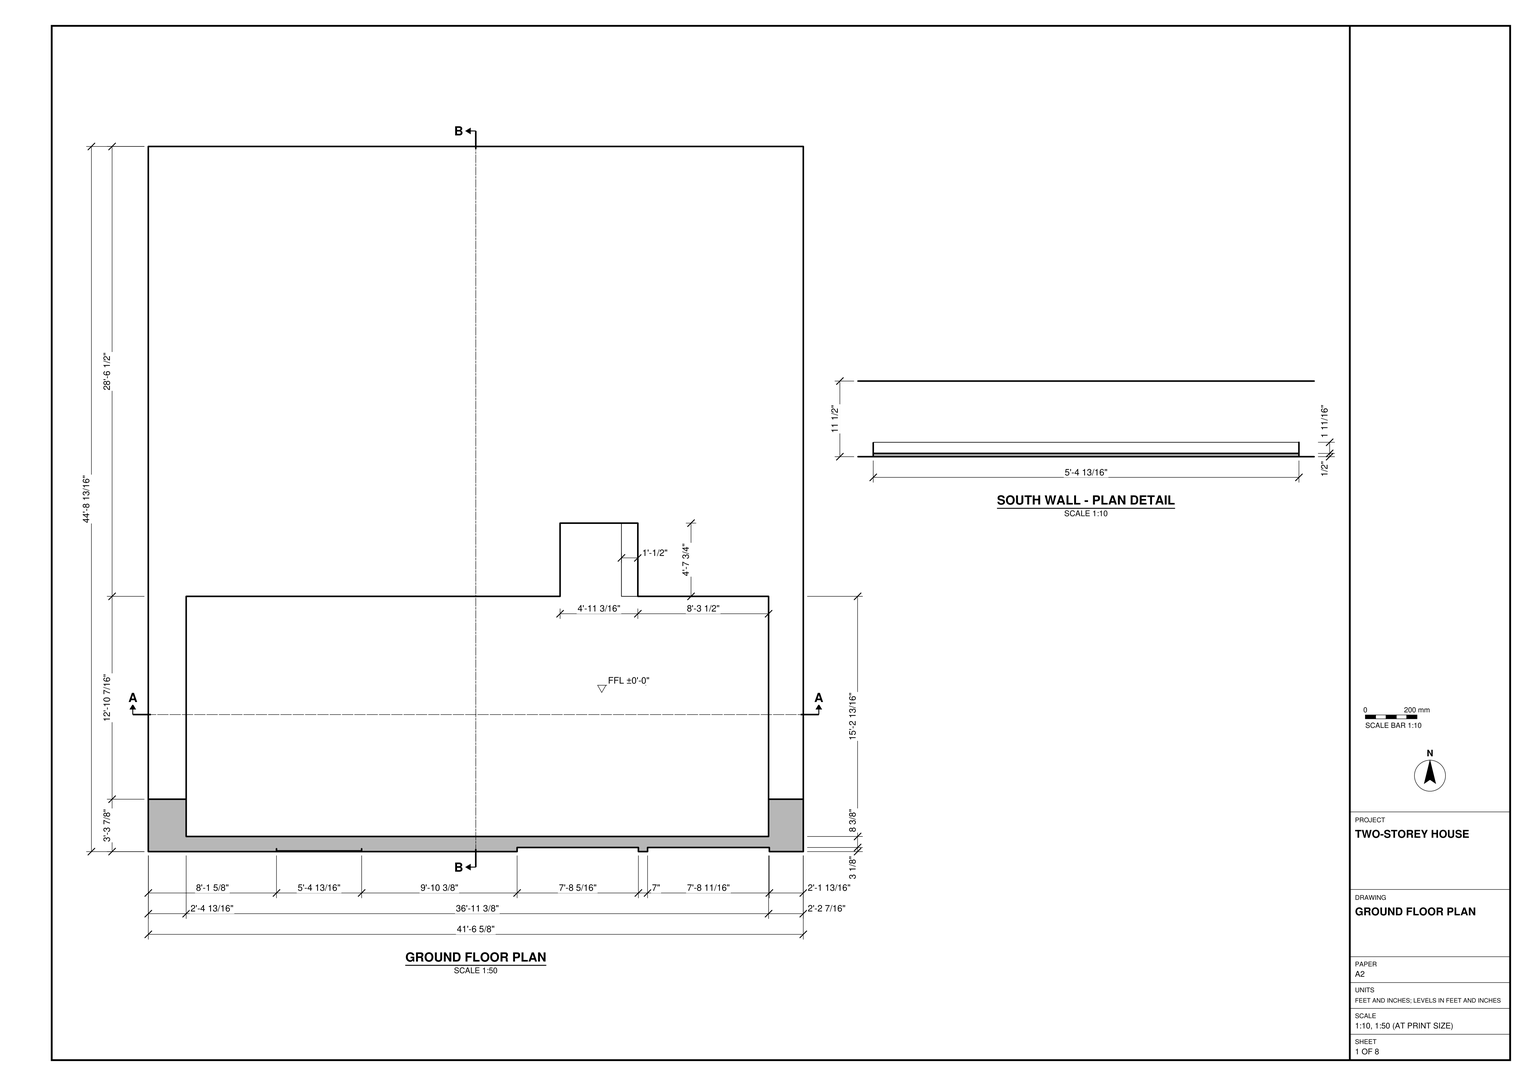
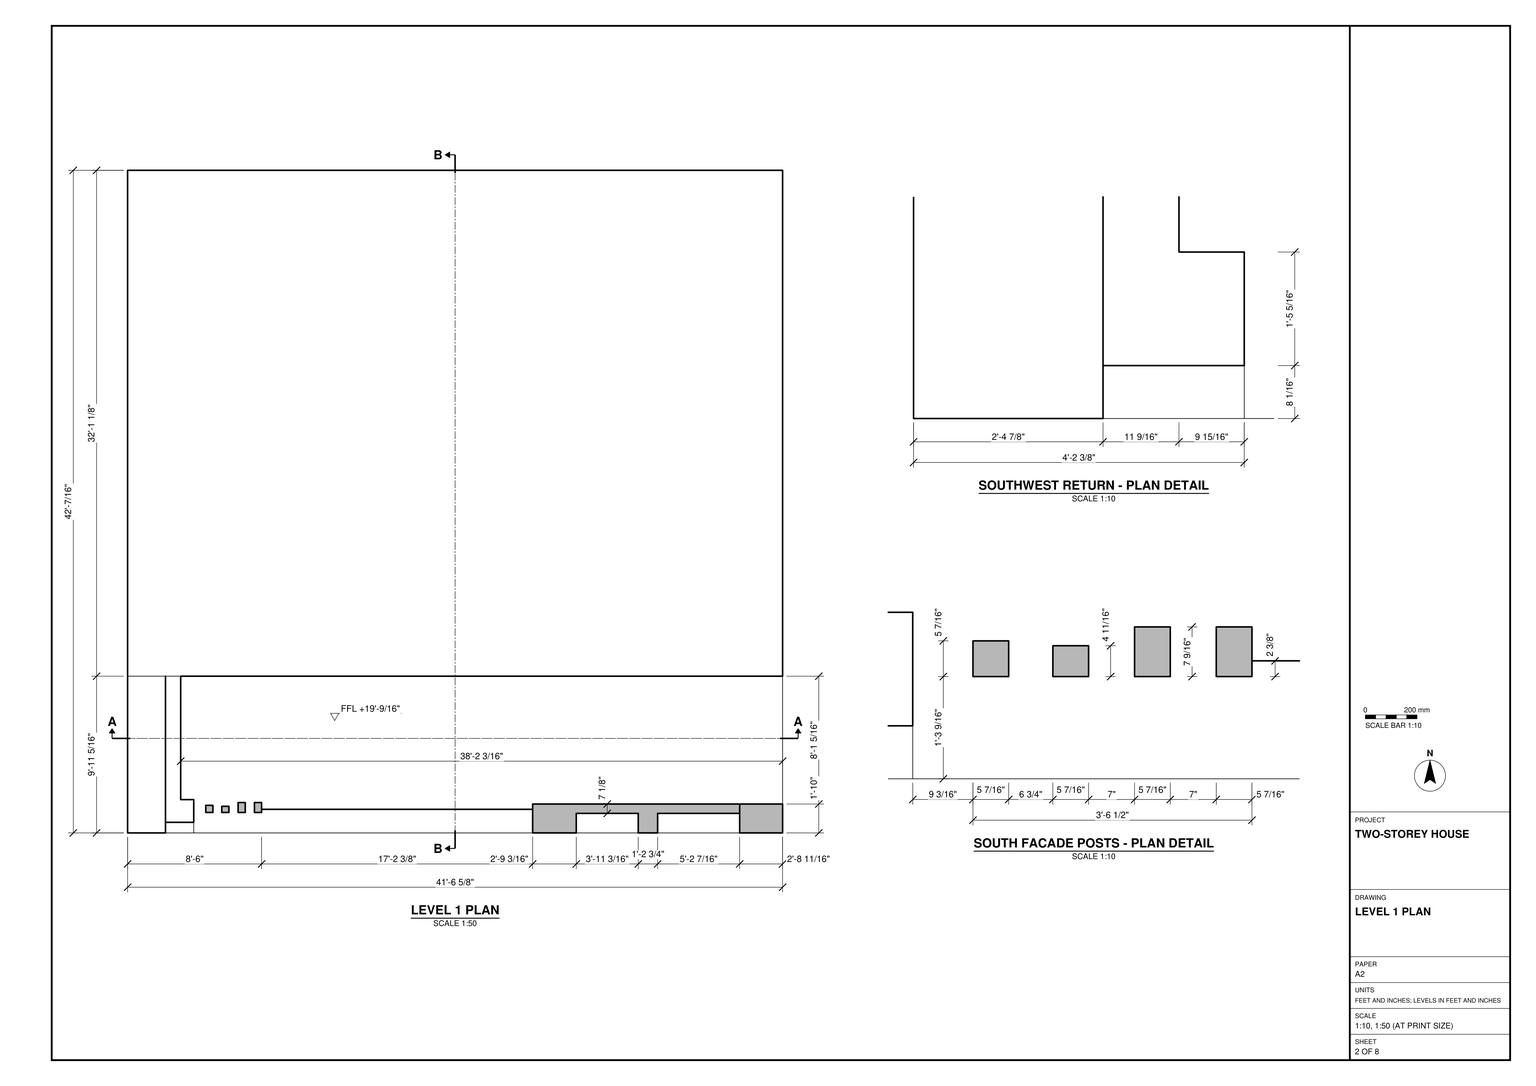
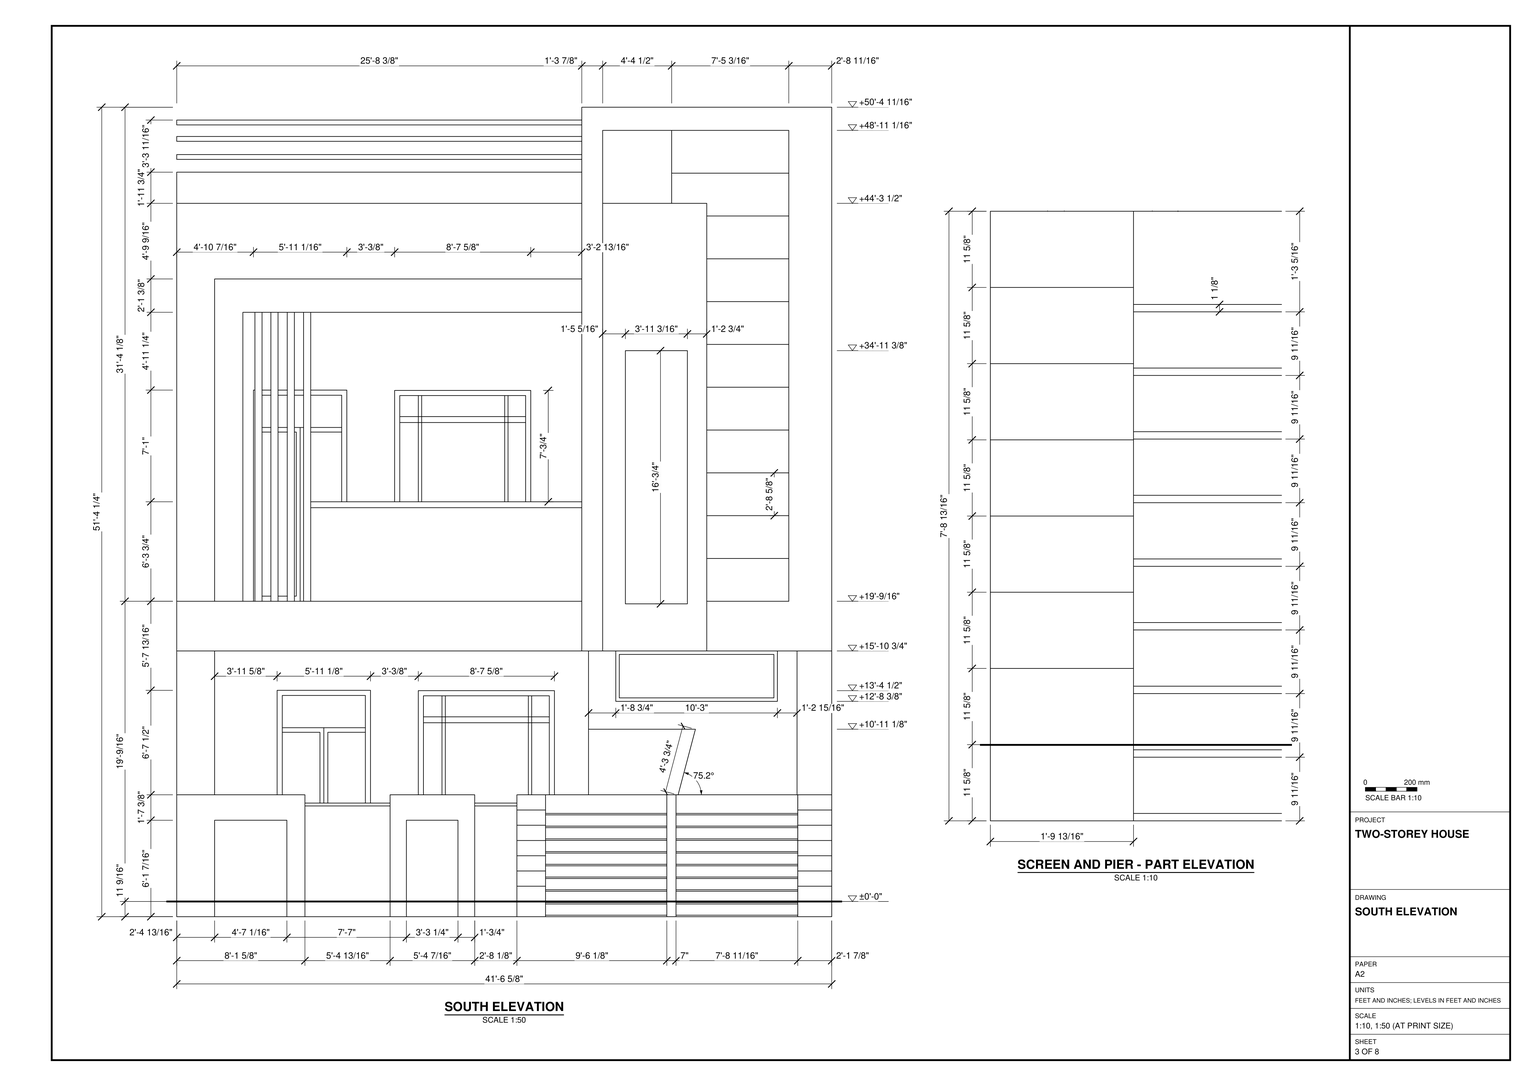
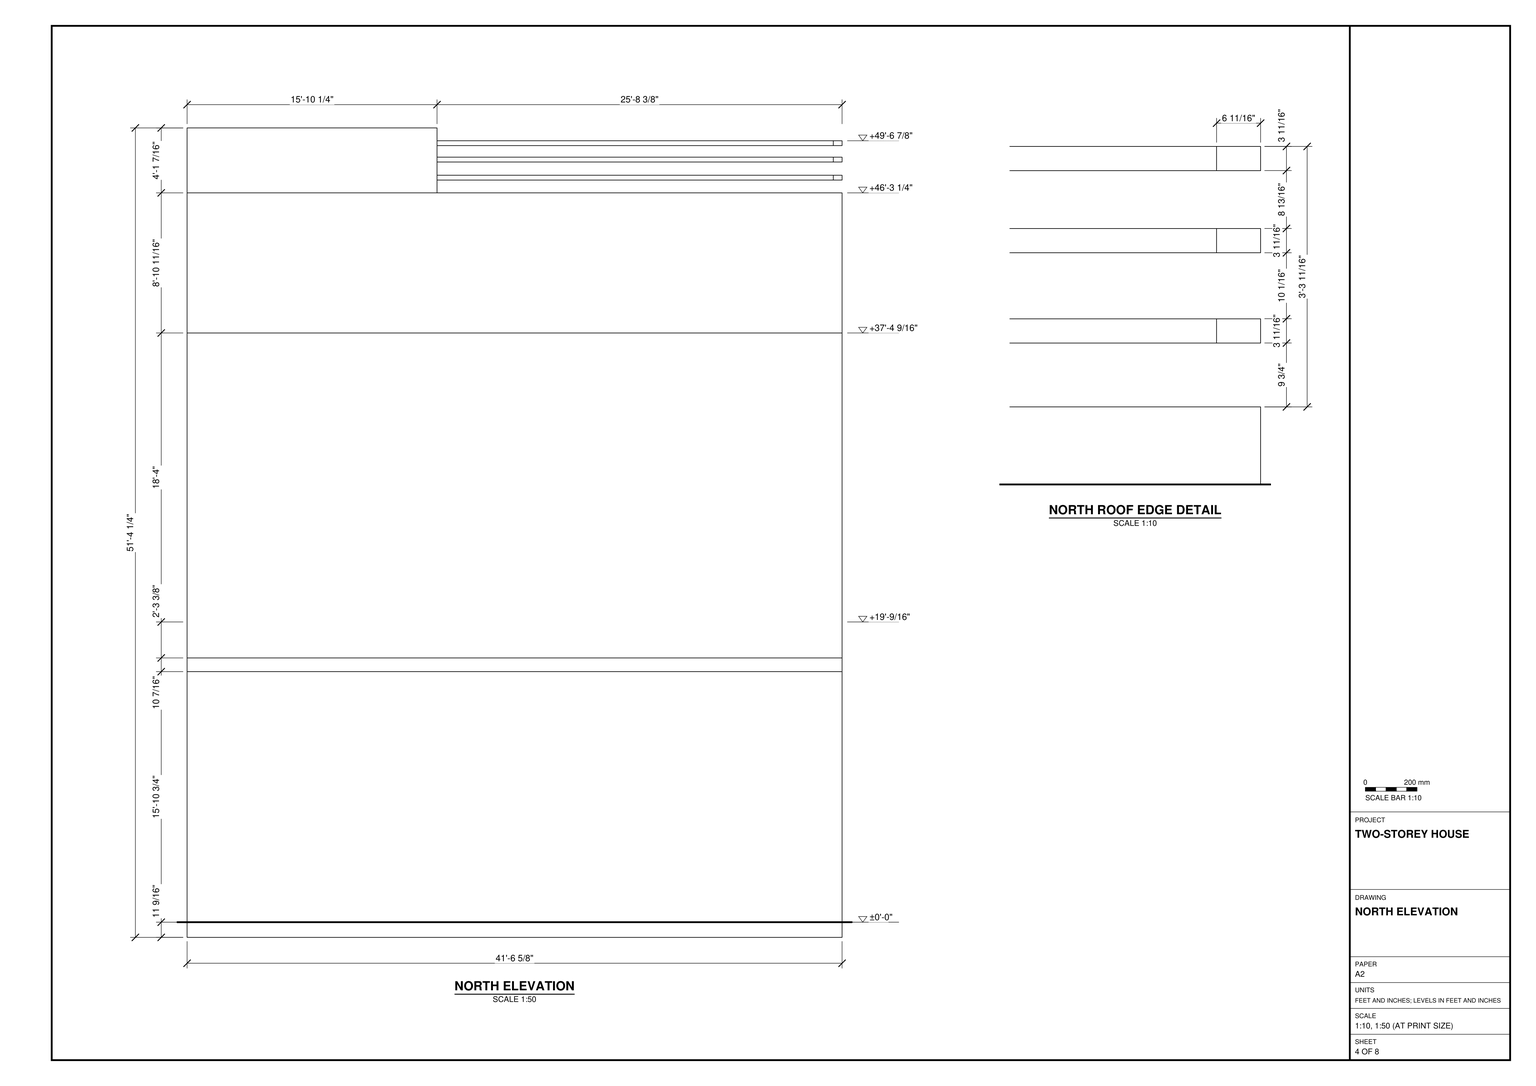
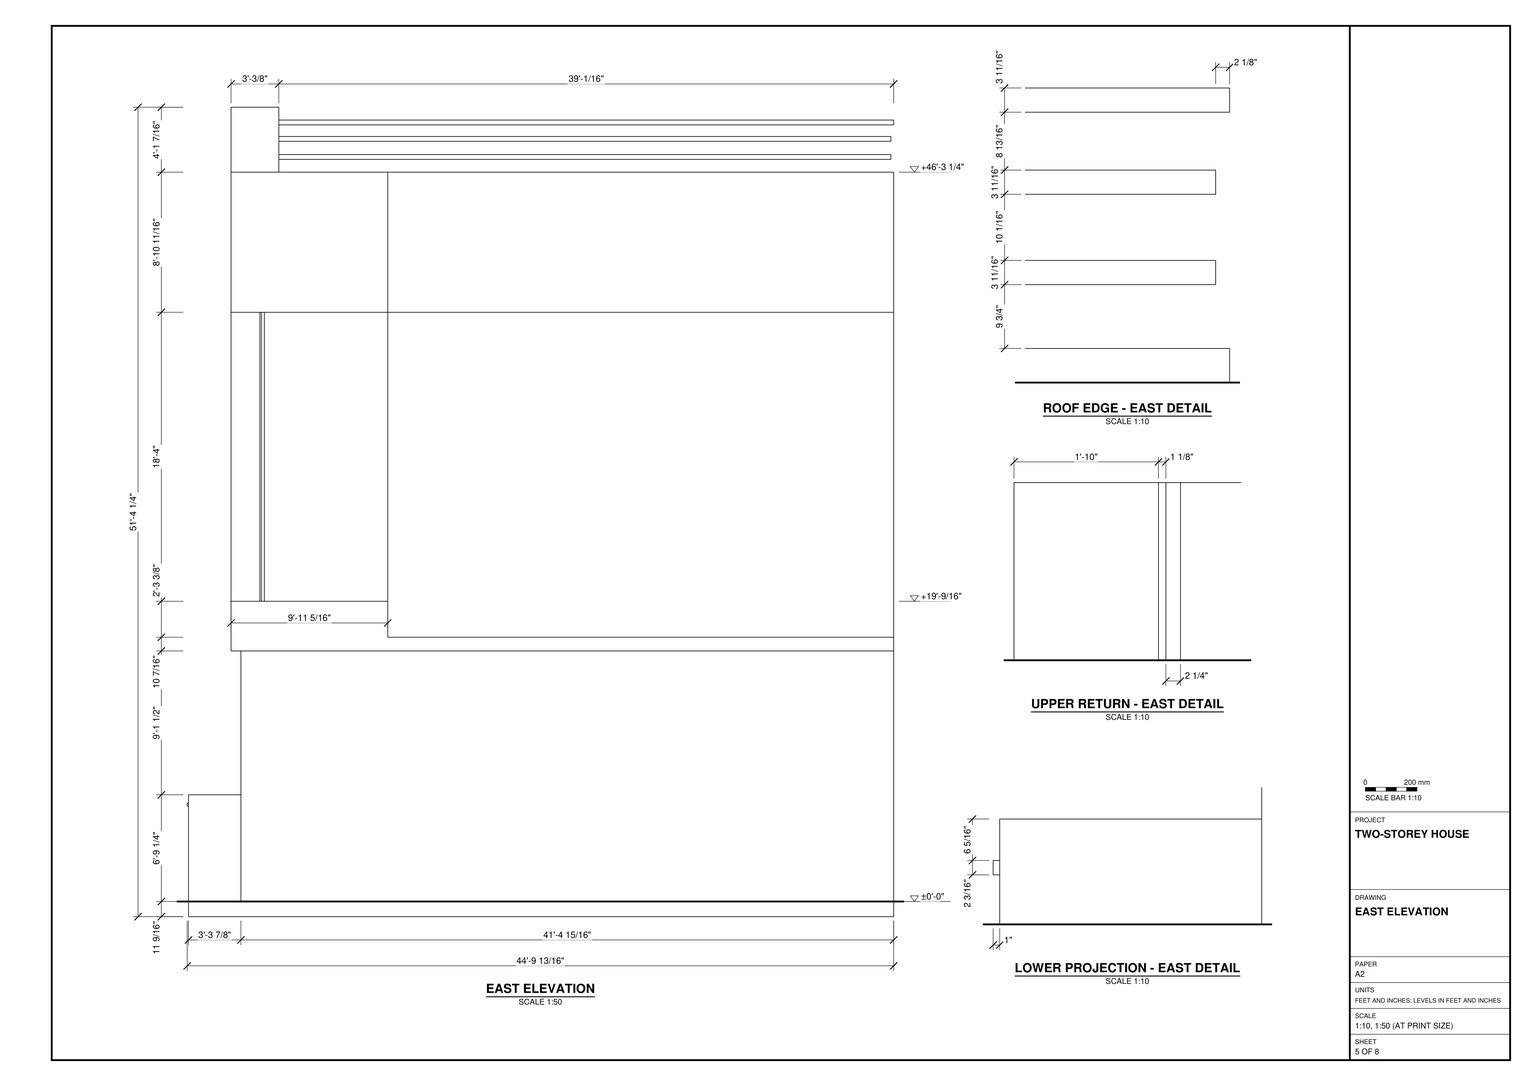
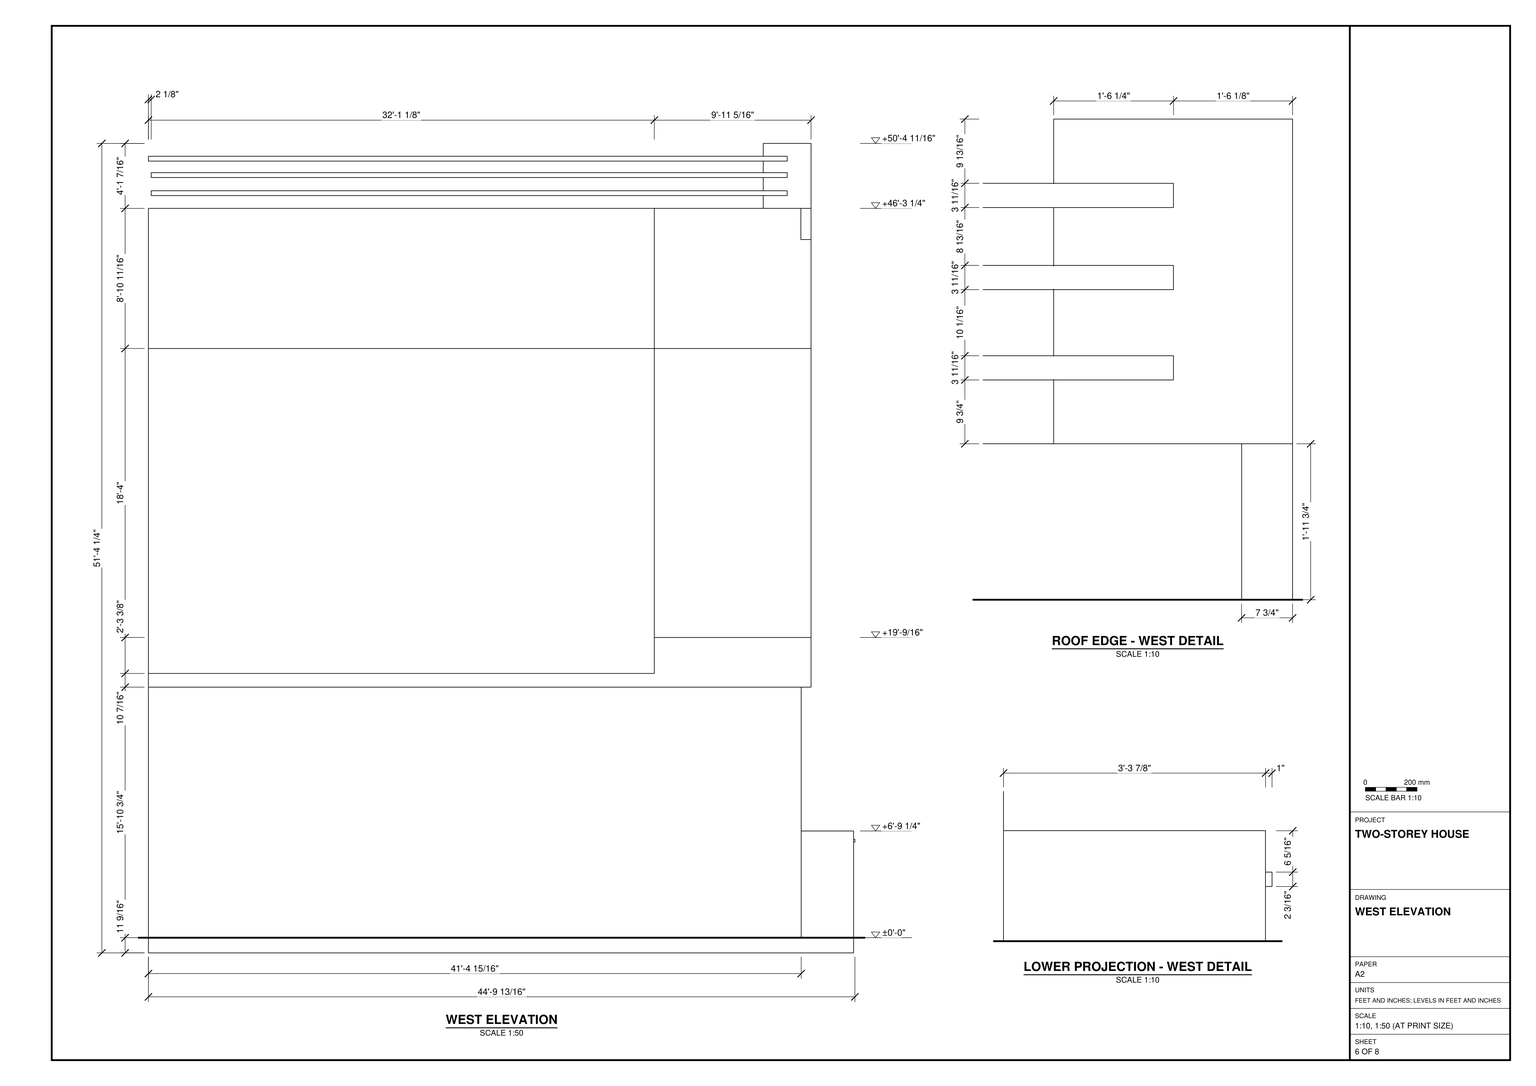
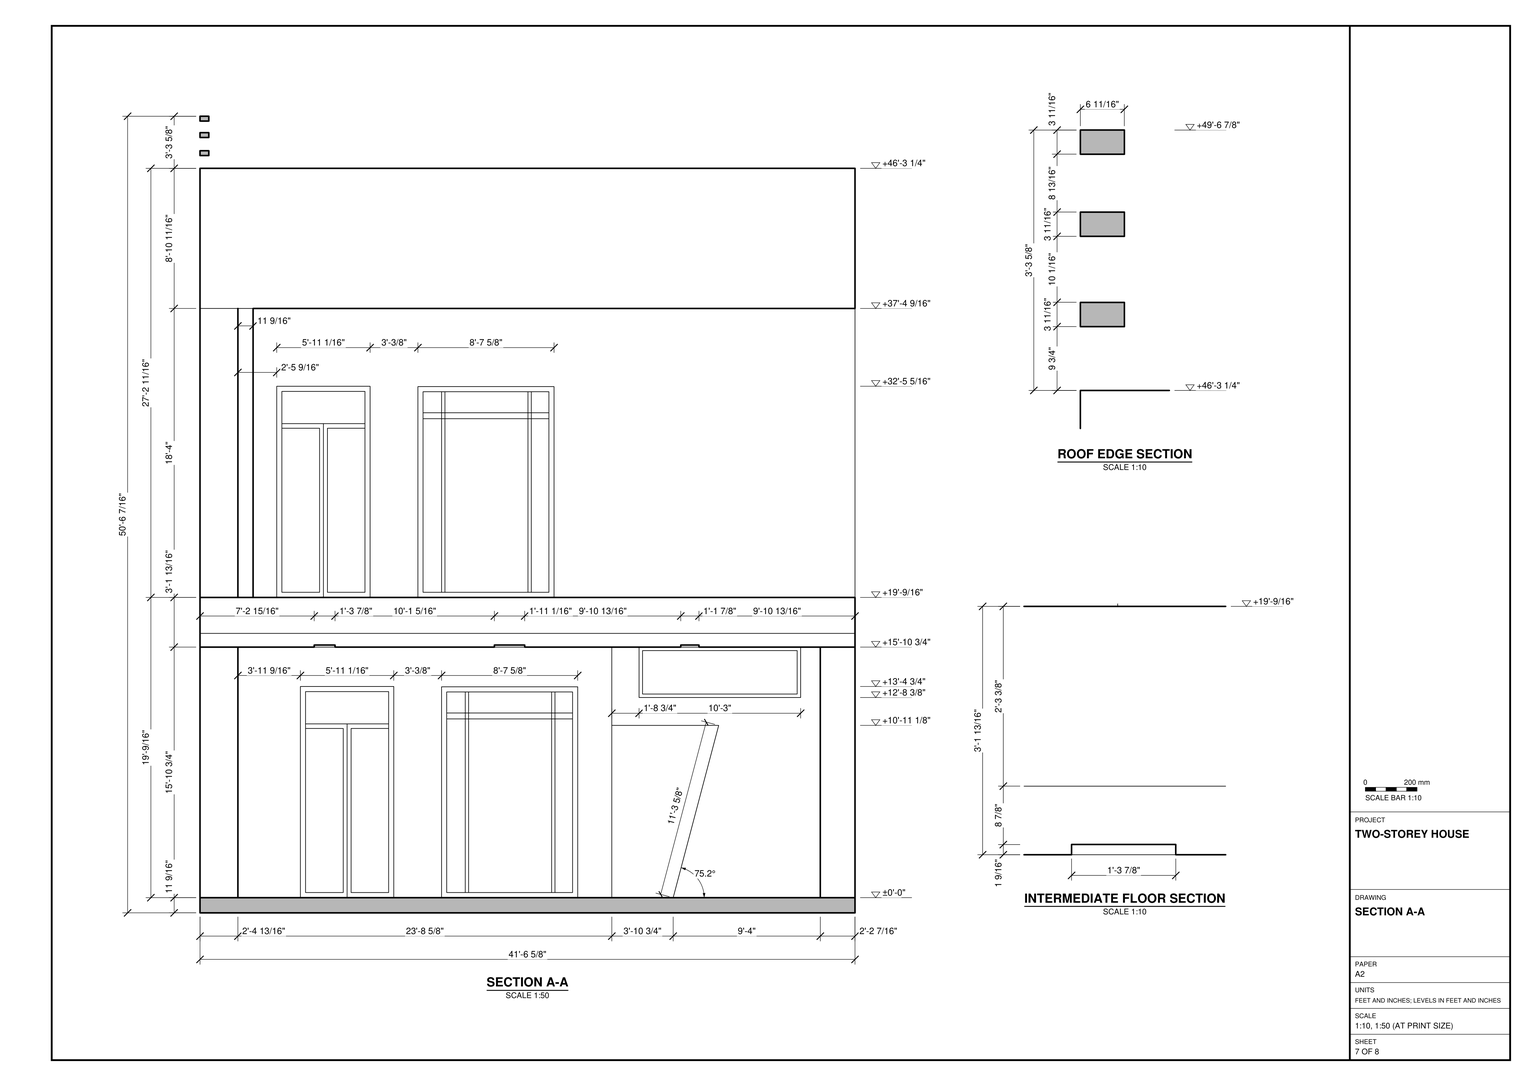
Build the two-storey house in SketchUp from task_files/diagram_01.pdf. Work in feet and inches. Set the overall width to 41'-6 5/8", depth to 44'-9 13/16" and height to 51'-4 1/4". Use ±0'-0" for the ground floor and +19'-9/16" for the upper floor.

Use the plans to lay out the slabs and walls at their drawn thicknesses. Preserve the setback between the house and the south boundary, the stepped ground-floor outline and the upper balcony with its southwest return. Use the south elevation to position the framed openings behind the balcony parapet and front boundary wall. Model the slender vertical posts at the west end of the balcony, the horizontal members at the roofline and the tall frame around the banded panel on the east side. At ground level, distinguish the solid portions of the boundary wall from the two slatted screen bays and their piers.

Follow the sheets for the roof and any stairs, built-in joinery or main furniture shown. Keep shell elements such as walls, slabs and roof separate as groups or components. Group each furniture or joinery piece separately and use components for repeated parts. Any decor or loose items shown may be suitable library components. Save one SketchUp model as output_files/two_storey_house_with_a_screened_south_balcony.skp.

# SketchUp Ruby script. Lengths in inches.
U = 1.inch
M = Sketchup.active_model
def pt(a) = Geom::Point3d.new(a.map { |v| v * U })
def face(e, loops, mat)
  f = e.add_face(loops[0].map { |a| pt(a) })
  loops[1..].each { |l| e.add_face(l.map { |a| pt(a) }).erase! }
  f.material = f.back_material = mat if mat
  f
end
# faces: each face lists its corners as indices into pts; further lists are holes
def faces(e, pts, list, mat = nil) = list.each { |f| face(e, (f[0].is_a?(Array) ? f : [f]).map { |l| l.map { |i| pts[i] } }, mat) }
# xy, xz, yz: faces in a plane at the given z, y or x. An outline is a flat list of corners, or four numbers for a rectangle; further outlines are holes
def ring(l) = l.size == 4 ? [[l[0], l[1]], [l[2], l[1]], [l[2], l[3]], [l[0], l[3]]] : l.each_slice(2).to_a
def flat(e, list, mat, &to3) = list.each { |f| face(e, (f[0].is_a?(Array) ? f : [f]).map { |l| ring(l).map { |u, v| to3.(u, v) } }, mat) }
def xy(e, z, list, mat = nil) = flat(e, list, mat) { |x, y| [x, y, z] }
def xz(e, y, list, mat = nil) = flat(e, list, mat) { |x, z| [x, y, z] }
def yz(e, x, list, mat = nil) = flat(e, list, mat) { |y, z| [x, y, z] }
def lines(e, pts, list) = list.each { |a, b| e.add_line(pt(pts[a]), pt(pts[b])) }
# prism: a flat outline (further loops are holes) pulled along v
def prism(e, loops, v, mat = nil)
  f = face(e, loops, mat); d = Geom::Vector3d.new(v.map { |x| x * U })
  f.pushpull(f.normal.samedirection?(d) ? d.length : -d.length)
end
def box(e, o, s, mat = nil) = prism(e, [[o, [o[0] + s[0], o[1], o[2]], [o[0] + s[0], o[1] + s[1], o[2]], [o[0], o[1] + s[1], o[2]]]], [0, 0, s[2]], mat)
def at(x, y, z, deg = 0) = Geom::Transformation.translation(pt([x, y, z])) * Geom::Transformation.rotation(ORIGIN, Z_AXIS, deg.degrees)
def axes(o, x, y, z) = Geom::Transformation.new([*x, 0, *y, 0, *z, 0, *pt(o).to_a, 1])
def part(name) = M.definitions.add(name)
# library, detail: a bought-in or finely detailed component or shape, given as its bounding box
def library(name, o, s) = part(name).tap { |d| box(d.entities, o, s) }
def detail(e, o, s) = box(e.add_group.entities, o, s)
def put(e, d, t, mat = nil) = e.add_instance(d, t).tap { |i| i.material = mat if mat }
def group(e, t, mat = nil) = e.add_group.tap { |g| g.transformation = t; g.material = mat if mat }.entities
root = M.entities
M.materials.add("[0131_Silver]").color = [192, 192, 192]
M.materials.add("[0134_DimGray]").color = [105, 105, 105]
M.materials.add("[Concrete Tile]").color = [203, 190, 164]
M.materials.add("[Encaustic Tile Circular 01]").color = [123, 123, 122]
M.materials.add("[Translucent Glass Tinted]").color = [8, 201, 241]
M.materials["[Translucent Glass Tinted]"].alpha = 0.48
M.materials.add("[Wood Bamboo]").color = [177, 105, 43]
M.materials.add("[Wood Cherry Original]").color = [152, 86, 42]
M.materials.add("[Wood Plywood Knots]").color = [137, 122, 41]
xy(root,0,[[0,1,0,537.8125,498.625,537.8125,498.625,1,472.79,1,472.75,4.125,380.08,4.125,380.08,1,373.09,1,373.09,4.125,280.76,4.125,280.76,1,162.41,1,162.41,3.1875,97.6,3.1875,97.6,1],[97.6,1,162.41,1.5],[97.6,1.5,162.41,3.1875]])
xy(root,11.5625,[[28.84,12.51,472.2,12.51,472.2,195.3125,360.2,195.3125,360.2,251.0625,313.48,251.0625,313.48,195.3125,28.84,195.3125],[0,40.89,0,537.8125,498.625,537.8125,498.625,40.89,472.2,40.89,472.2,195.3125,360.2,195.3125,360.2,251.0625,313.48,251.0625,313.48,195.3125,28.84,195.3125,28.84,40.89]])
xy(root,84.3125,[[97.6,1,162.41,1.5],[226.83,1,258.97,12.51],[97.6,1.5,162.41,3.1875],[97.6,12.51,162.41,40.89],[226.83,12.51,258.97,40.89]])
xy(root,84.3125,[[97.6,0,162.41,1],[226.83,0,258.97,1]],"[0131_Silver]")
xy(root,86.5,[[97.6,0,162.41,40.89],[226.83,0,258.97,40.89]],"[0131_Silver]")
xy(root,92.8125,[[0,1,97.6,1,97.6,12.51,28.84,12.51,28.84,40.89,0,40.89],[162.41,1,226.83,12.51],[258.97,1,280.76,12.51],[373.09,1,380.08,1,380.08,4.125,472.75,4.125,472.2,40.89,472.2,12.51,280.76,12.51,280.76,4.125,373.09,4.125],[472.79,1,498.625,1,498.625,40.89,472.2,40.89,472.75,4.125]])
xy(root,142.72,[[313.48,195.3125,394.85,251.0625]])
xy(root,202.3125,[[[0,33.375,0,40.89,28.84,40.89,28.84,195.3125,472.2,195.3125,472.2,40.89,498.625,40.89,498.625,33.375],[235.64,82.58,239.36,83.07,242.83,84.5,245.8,86.79,248.09,89.76,249.52,93.23,250.01,96.95,249.52,100.67,248.09,104.14,245.8,107.12,242.83,109.4,239.36,110.84,235.64,111.33,231.92,110.84,228.45,109.4,225.47,107.12,223.1875,104.14,221.75,100.67,221.26,96.95,221.75,93.23,223.1875,89.76,225.47,86.79,228.45,84.5,231.92,83.07],[94.86,85.39,97.85,85.78,100.64,86.9375,103.04,88.78,104.87,91.17,106.03,93.96,106.42,96.95,106.03,99.94,104.87,102.73,103.04,105.13,100.64,106.96,97.85,108.12,94.86,108.51,91.87,108.12,89.08,106.96,86.68,105.13,84.85,102.73,83.69,99.94,83.3,96.95,83.69,93.96,84.85,91.17,86.68,88.78,89.08,86.9375,91.87,85.78],[372.91,86,375.74,86.38,378.38,87.47,380.65,89.21,382.39,91.48,383.48,94.12,383.86,96.95,383.48,99.78,382.39,102.42,380.65,104.69,378.38,106.43,375.74,107.52,372.91,107.9,370.08,107.52,367.4375,106.43,365.17,104.69,363.43,102.42,362.34,99.78,361.96,96.95,362.34,94.12,363.43,91.48,365.17,89.21,367.4375,87.47,370.08,86.38]],[0,40.89,0,537.8125,498.625,537.8125,498.625,40.89,472.2,40.89,472.2,195.3125,28.84,195.3125,28.84,40.89]])
xy(root,203.875,[[235.64,82.58,231.92,83.07,228.45,84.5,225.47,86.79,223.1875,89.76,221.75,93.23,221.26,96.95,221.75,100.67,223.1875,104.14,225.47,107.12,228.45,109.4,231.92,110.84,235.64,111.33,239.36,110.84,242.83,109.4,245.8,107.12,248.09,104.14,249.52,100.67,250.01,96.95,249.52,93.23,248.09,89.76,245.8,86.79,242.83,84.5,239.36,83.07],[94.86,85.39,91.87,85.78,89.08,86.9375,86.68,88.78,84.85,91.17,83.69,93.96,83.3,96.95,83.69,99.94,84.85,102.73,86.68,105.13,89.08,106.96,91.87,108.12,94.86,108.51,97.85,108.12,100.64,106.96,103.04,105.13,104.87,102.73,106.03,99.94,106.42,96.95,106.03,93.96,104.87,91.17,103.04,88.78,100.64,86.9375,97.85,85.78],[372.91,86,370.08,86.38,367.4375,87.47,365.17,89.21,363.43,91.48,362.34,94.12,361.96,96.95,362.34,99.78,363.43,102.42,365.17,104.69,367.4375,106.43,370.08,107.52,372.91,107.9,375.74,107.52,378.38,106.43,380.65,104.69,382.39,102.42,383.48,99.78,383.86,96.95,383.48,94.12,382.39,91.48,380.65,89.21,378.38,87.47,375.74,86.38]])
xy(root,212.75,[[0,152.6875,498.625,537.8125]])
xy(root,238.17,[[341.54,33.375,388.73,48.25]])
xy(root,240.125,[[0,33.375,28.85,152.6875],[28.85,33.375,50.35,41.4375],[[50.35,33.375,308.35,33.375,308.35,55.375,498.625,55.375,498.625,152.6875,40.41,152.6875,40.41,58.72,50.35,58.72],[59.52,48.9375,64.95,54.375],[71.68,48.9375,77.12,53.63]],[403.49,33.375,465.94,48.25],[28.85,41.4375,50.35,41.4375,50.35,58.72,40.41,58.72,40.41,152.6875,28.85,152.6875],
  [403.49,48.25,465.94,55.375],[84.12,48.9375,89.56,56.5],[96.56,48.9375,101.99,56.5]])
xy(root,311.375,[[101.99,48.9375,308.35,51.33],[101.99,51.33,308.35,53.73]])
xy(root,315.875,[[101.99,48.9375,308.35,53.73]],"[Wood Plywood Knots]")
xy(root,430.92,[[341.54,33.375,388.73,48.25]])
xy(root,460.125,[[[50.35,41.4375,50.35,58.72,40.41,58.72,40.41,152.6875,498.625,152.6875,498.625,55.375,308.35,55.375,308.35,41.4375],[122.01,89.4375,123.91,89.6875,125.67,90.42,127.18,91.58,128.35,93.09,129.08,94.86,129.33,96.75,129.08,98.64,128.35,100.41,127.18,101.92,125.67,103.08,123.91,103.8125,122.01,104.0625,120.12,103.8125,118.36,103.08,116.84,101.92,115.68,100.41,114.95,98.64,114.7,96.75,114.95,94.86,115.68,93.09,116.84,91.58,118.36,90.42,120.12,89.6875],[260.75,91,262.24,91.2,263.63,91.77,264.82,92.68,265.73,93.875,266.31,95.26,266.5,96.75,266.31,98.24,265.73,99.625,264.82,100.82,263.63,101.73,262.24,102.3,260.75,102.5,259.27,102.3,257.88,101.73,256.6875,100.82,255.77,99.625,255.2,98.24,255,96.75,255.2,95.26,255.77,93.875,256.6875,92.68,257.88,91.77,259.27,91.2],[59.52,48.9375,64.95,54.375],[71.68,48.9375,77.12,53.63]],[84.12,48.9375,89.56,56.5],[96.56,48.9375,101.99,56.5],[0,152.6875,498.625,537.8125]])
xy(root,461.6875,[[122.01,89.4375,120.12,89.6875,118.36,90.42,116.84,91.58,115.68,93.09,114.95,94.86,114.7,96.75,114.95,98.64,115.68,100.41,116.84,101.92,118.36,103.08,120.12,103.8125,122.01,104.0625,123.91,103.8125,125.67,103.08,127.18,101.92,128.35,100.41,129.08,98.64,129.33,96.75,129.08,94.86,128.35,93.09,127.18,91.58,125.67,90.42,123.91,89.6875],[260.75,91,259.27,91.2,257.88,91.77,256.6875,92.68,255.77,93.875,255.2,95.26,255,96.75,255.2,98.24,255.77,99.625,256.6875,100.82,257.88,101.73,259.27,102.3,260.75,102.5,262.24,102.3,263.63,101.73,264.82,100.82,265.73,99.625,266.31,98.24,266.5,96.75,266.31,95.26,265.73,93.875,264.82,92.68,263.63,91.77,262.24,91.2]])
xy(root,485.51,[[28.85,33.375,308.35,41.4375]])
xy(root,543.07,[[0,33.375,308.35,41.125],[324.24,33.375,376.76,48.25],[376.76,33.375,403.49,48.25]])
xy(root,566.8125,[[0,41.125,308.35,41.125,308.35,69.75,498.625,69.75,498.625,152.6875,0,152.6875],[0,152.6875,498.625,537.8125]])
xy(root,576.53,[[0,51.51,0,535.6875,6.71,535.6875,6.71,55.2,308.35,55.2,308.35,51.51]],"[0134_DimGray]")
xy(root,580.22,[[0,51.51,308.35,51.51,308.35,55.2,6.71,55.2,6.71,535.6875,0,535.6875]],"[0134_DimGray]")
xy(root,590.28,[[0,51.51,0,535.6875,6.71,535.6875,6.71,55.2,308.35,55.2,308.35,51.51]],"[0134_DimGray]")
xy(root,593.97,[[0,51.51,308.35,51.51,308.35,55.2,6.71,55.2,6.71,535.6875,0,535.6875]],"[0134_DimGray]")
xy(root,598.625,[[324.24,33.375,376.76,48.25],[376.76,33.375,465.94,48.25]])
xy(root,602.78,[[0,51.51,0,537.8125,6.71,537.8125,6.71,55.2,308.35,55.2,308.35,51.51]],"[0134_DimGray]")
xy(root,606.47,[[0,51.51,308.35,51.51,308.35,55.2,6.71,55.2,6.71,537.8125,0,537.8125]],"[0134_DimGray]")
xy(root,616.25,[[308.35,33.375,498.625,69.75]])
xz(root,0,[[97.6,84.3125,162.41,86.5],[226.83,84.3125,258.97,86.5]],"[0131_Silver]")
xz(root,1,[[28.84,0,83.84,73.4375],[97.6,0,162.41,84.3125],[174.83,0,214.08,73.4375],[226.83,0,258.97,84.3125]])
xz(root,1,[[0,0,28.84,0,28.84,73.4375,83.84,73.4375,83.84,0,97.6,0,97.6,92.8125,0,92.8125],[162.41,0,174.83,0,174.83,73.4375,214.08,73.4375,214.08,0,226.83,0,226.83,92.8125,162.41,92.8125],[258.97,0,280.76,11.6],[373.09,0,380.08,92.8125],[472.79,0,498.625,11.6],
  [258.97,11.6,280.76,23.2],[472.79,11.6,498.625,23.2],[258.97,23.2,280.76,34.8],[472.79,23.2,498.625,34.8],[258.97,34.8,280.76,46.41],
  [472.79,34.8,498.625,46.41],[258.97,46.41,280.76,58.01],[472.79,46.41,498.625,58.01],[258.97,58.01,280.76,69.61],[472.79,58.01,498.625,69.61],
  [258.97,69.61,280.76,81.21],[472.79,69.61,498.625,81.21],[258.97,81.21,280.76,92.8125],[472.79,81.21,498.625,92.8125]],"[Concrete Tile]")
xz(root,1.5,[[97.6,0,162.41,84.3125]])
xz(root,4.125,[[280.76,0,373.09,1.125],[380.08,0,472.75,1.125],[280.76,9.6875,373.09,10.8125],[380.08,9.6875,472.75,10.8125],[280.76,19.375,373.09,20.5],
  [380.08,19.375,472.75,20.5],[280.76,29.0625,373.09,30.1875],[380.08,29.0625,472.75,30.1875],[280.76,38.75,373.09,39.875],[380.08,38.75,472.75,39.875],
  [280.76,48.4375,373.09,49.5625],[380.08,48.4375,472.75,49.5625],[280.76,58.125,373.09,59.25],[380.08,58.125,472.75,59.25],[280.76,67.8125,373.09,68.9375],
  [380.08,67.8125,472.75,68.9375],[280.76,77.5,373.09,78.625],[380.08,77.5,472.75,78.625]])
xz(root,4.125,[[280.76,1.125,373.09,9.6875],[380.08,1.125,472.75,9.6875],[280.76,10.8125,373.09,19.375],[380.08,10.8125,472.75,19.375],[280.76,20.5,373.09,29.0625],
  [380.08,20.5,472.75,29.0625],[280.76,30.1875,373.09,38.75],[380.08,30.1875,472.75,38.75],[280.76,39.875,373.09,48.4375],[380.08,39.875,472.75,48.4375],
  [280.76,49.5625,373.09,58.125],[380.08,49.5625,472.75,58.125],[280.76,59.25,373.09,67.8125],[380.08,59.25,472.75,67.8125],[280.76,68.9375,373.09,77.5],
  [380.08,68.9375,472.75,77.5],[280.76,78.625,373.09,92.8125],[380.08,78.625,472.75,92.8125]],"[Wood Cherry Original]")
xz(root,12.51,[[28.84,11.5625,28.84,92.8125,97.6,92.8125,97.6,84.3125,162.41,84.3125,162.41,92.8125,226.83,92.8125,226.83,84.3125,258.97,84.3125,258.97,92.8125,472.2,92.8125,472.2,11.5625]])
xz(root,33.375,[[308.35,202.3125,324.24,202.3125,324.24,598.625,465.94,598.625,465.94,240.125,403.49,240.125,403.49,202.3125,498.625,202.3125,498.625,616.25,308.35,616.25]],"[0131_Silver]")
xz(root,33.375,[[0,202.3125,308.35,240.125],[[324.24,202.3125,403.49,543.07],[341.54,238.17,388.73,430.92]],[0,240.125,28.85,240.125,28.85,485.51,308.35,485.51,308.35,543.07,0,543.07]],"[0134_DimGray]")
xz(root,40.89,[[0,11.5625,28.84,92.8125],[472.2,11.5625,498.625,92.8125],[97.6,84.3125,162.41,86.5],[226.83,84.3125,258.97,86.5],[0,92.8125,28.84,202.3125],
  [472.2,92.8125,498.625,202.3125]])
xz(root,41.125,[[0,543.07,308.35,566.8125]])
xz(root,41.4375,[[28.85,240.125,50.35,240.125,50.35,460.125,308.35,460.125,308.35,485.51,28.85,485.51]])
xz(root,48.25,[[403.49,240.125,465.94,272.72],[403.49,272.72,465.94,305.31],[403.49,305.31,465.94,337.9],[403.49,337.9,465.94,370.49],[403.49,370.49,465.94,403.08],
  [403.49,403.08,465.94,435.67],[403.49,435.67,465.94,468.26],[403.49,468.26,465.94,500.85],[403.49,500.85,465.94,533.44],[403.49,533.44,465.94,533.44,465.94,566.03,376.76,566.03,376.76,543.07,403.49,543.07],
  [376.76,566.03,465.94,598.625]])
xz(root,48.25,[[341.54,238.17,388.73,430.92],[324.24,543.07,376.76,598.625]],"[Encaustic Tile Circular 01]")
xz(root,48.9375,[[59.52,240.125,64.95,460.125],[71.68,240.125,77.12,460.125],[84.12,240.125,89.56,460.125],[96.56,240.125,101.99,460.125]],"[Wood Bamboo]")
xz(root,48.9375,[[101.99,311.375,308.35,315.875]],"[Wood Plywood Knots]")
xz(root,51.33,[[101.99,240.125,308.35,311.375]],"[Translucent Glass Tinted]")
xz(root,51.51,[[0,576.53,308.35,580.22],[0,590.28,308.35,593.97],[0,602.78,308.35,606.47]],"[0134_DimGray]")
xz(root,53.63,[[71.68,240.125,77.12,460.125]])
xz(root,53.73,[[101.99,311.375,308.35,315.875]])
xz(root,54.375,[[59.52,240.125,64.95,460.125]])
xz(root,55.2,[[6.71,576.53,308.35,580.22],[6.71,590.28,308.35,593.97],[6.71,602.78,308.35,606.47]],"[0134_DimGray]")
xz(root,55.375,[[308.35,240.125,465.94,460.125],[465.94,240.125,498.625,460.125]])
xz(root,56.5,[[84.12,240.125,89.56,460.125],[96.56,240.125,101.99,460.125]])
xz(root,58.72,[[40.41,240.125,50.35,460.125]])
xz(root,69.75,[[308.35,566.8125,498.625,616.25]])
xz(root,152.6875,[[0,212.75,498.625,240.125],[40.41,240.125,58.42,240.125,58.42,400.9,129.49,400.9,129.49,240.125,165.88,240.125,165.88,400.65,269.52,400.65,269.52,240.125,498.625,240.125,498.625,460.125,40.41,460.125],[62.33,244.03,91.02,368.95],[97.02,244.03,125.58,368.95],[169.79,244.03,183.92,376.21],
  [252.21,244.03,265.61,376.21],[62.33,372.45,125.58,397],[169.79,380.72,183.92,396.74],[186.46,380.72,249.67,396.74],[252.21,380.72,265.61,396.74],
  [0,460.125,498.625,566.8125]])
xz(root,152.6875,[[58.42,240.125,93.96,240.125,93.96,372.45,62.33,372.45,62.33,368.95,91.02,368.95,91.02,244.03,62.33,244.03,62.33,397,125.58,397,125.58,244.03,97.02,244.03,97.02,368.95,125.58,368.95,125.58,372.45,93.96,372.45,93.96,240.125,129.49,240.125,129.49,400.9,58.42,400.9],[[165.88,240.125,269.52,400.65],[169.79,244.03,265.61,396.74]],[183.92,244.03,186.46,376.21],[186.46,244.03,249.67,376.21],[249.67,244.03,252.21,376.21],
  [169.79,376.21,183.92,380.72],[183.92,376.21,186.46,380.72],[186.46,376.21,249.67,380.72],[249.67,376.21,252.21,380.72],[252.21,376.21,265.61,380.72],
  [183.92,380.72,186.46,396.74],[249.67,380.72,252.21,396.74]],"[Wood Cherry Original]")
xz(root,195.3125,[[28.84,11.5625,76.43,11.5625,76.43,172.34,147.51,172.34,147.51,11.5625,183.89,11.5625,183.89,172.09,287.53,172.09,287.53,11.5625,313.48,11.5625,313.48,202.3125,28.84,202.3125],[360.2,11.5625,472.2,11.5625,472.2,202.3125,457.24,202.3125,457.24,163.9375,334.24,163.9375,334.24,202.3125,313.48,202.3125,313.48,142.72,394.85,142.72],[80.34,15.47,109.03,140.38],[115.03,15.47,143.6,140.38],[187.8,15.47,201.93,147.65],
  [270.22,15.47,283.62,147.65],[80.34,143.88,143.6,168.43],[187.8,152.15,201.93,168.18],[204.47,152.15,267.68,168.18],[270.22,152.15,283.62,168.18],
  [[334.24,163.9375,457.24,202.3125],[336.89,166.59,454.59,199.66]],[336.89,166.59,454.59,199.66]])
xz(root,195.3125,[[76.43,11.5625,111.97,11.5625,111.97,143.88,80.34,143.88,80.34,140.38,109.03,140.38,109.03,15.47,80.34,15.47,80.34,168.43,143.6,168.43,143.6,15.47,115.03,15.47,115.03,140.38,143.6,140.38,143.6,143.88,111.97,143.88,111.97,11.5625,147.51,11.5625,147.51,172.34,76.43,172.34],[[183.89,11.5625,287.53,172.09],[187.8,15.47,283.62,168.18]],[201.93,15.47,204.47,147.65],[204.47,15.47,267.68,147.65],[267.68,15.47,270.22,147.65],
  [187.8,147.65,201.93,152.15],[201.93,147.65,204.47,152.15],[204.47,147.65,267.68,152.15],[267.68,147.65,270.22,152.15],[270.22,147.65,283.62,152.15],
  [201.93,152.15,204.47,168.18],[267.68,152.15,270.22,168.18]],"[Wood Cherry Original]")
xz(root,251.0625,[[313.48,11.5625,360.2,11.5625,394.85,142.72,313.48,142.72]])
xz(root,535.6875,[[0,576.53,6.71,580.22],[0,590.28,6.71,593.97]])
xz(root,537.8125,[[0,0,498.625,11.5625],[0,11.5625,498.625,202.3125],[0,202.3125,498.625,212.75],[0,212.75,498.625,460.125],[0,460.125,498.625,566.8125],
  [0,602.78,6.71,606.47]])
yz(root,0,[[1,0,1,92.8125,40.89,92.8125,40.89,11.5625,537.8125,11.5625,537.8125,0],[40.89,11.5625,537.8125,202.3125],[33.375,202.3125,33.375,240.125,152.6875,240.125,152.6875,212.75,537.8125,212.75,537.8125,202.3125],[152.6875,212.75,537.8125,460.125],[33.375,240.125,152.6875,460.125],
  [33.375,460.125,33.375,543.07,41.125,543.07,41.125,566.8125,152.6875,566.8125,152.6875,460.125],[152.6875,460.125,537.8125,566.8125]])
yz(root,0,[[51.51,576.53,535.6875,580.22],[51.51,590.28,535.6875,593.97],[51.51,602.78,537.8125,606.47]],"[0134_DimGray]")
yz(root,6.71,[[55.2,576.53,535.6875,580.22],[55.2,590.28,535.6875,593.97],[55.2,602.78,537.8125,606.47]],"[0134_DimGray]")
yz(root,28.84,[[12.51,11.5625,40.89,92.8125],[40.89,11.5625,195.3125,202.3125]])
yz(root,28.85,[[33.375,240.125,41.4375,460.125],[41.4375,240.125,152.6875,460.125],[33.375,460.125,41.4375,485.51]])
yz(root,40.41,[[58.72,240.125,152.6875,460.125]])
yz(root,50.35,[[41.4375,240.125,58.72,460.125]])
yz(root,59.52,[[48.9375,240.125,54.375,460.125]],"[Wood Bamboo]")
yz(root,64.95,[[48.9375,240.125,54.375,460.125]],"[Wood Bamboo]")
yz(root,71.68,[[48.9375,240.125,53.63,460.125]],"[Wood Bamboo]")
yz(root,77.12,[[48.9375,240.125,53.63,460.125]],"[Wood Bamboo]")
yz(root,84.12,[[48.9375,240.125,56.5,460.125]],"[Wood Bamboo]")
yz(root,89.56,[[48.9375,240.125,56.5,460.125]],"[Wood Bamboo]")
yz(root,96.56,[[48.9375,240.125,56.5,460.125]],"[Wood Bamboo]")
yz(root,97.6,[[1,0,1.5,84.3125],[1.5,0,3.1875,84.3125],[0,84.3125,1,86.5],[1,84.3125,12.51,86.5],[12.51,84.3125,40.89,86.5],
  [1,86.5,12.51,92.8125]])
yz(root,101.99,[[48.9375,240.125,51.33,311.375]])
yz(root,101.99,[[51.33,240.125,56.5,240.125,56.5,460.125,48.9375,460.125,48.9375,315.875,53.73,315.875,53.73,311.375,51.33,311.375]],"[Wood Bamboo]")
yz(root,162.41,[[1,0,1.5,84.3125],[1.5,0,3.1875,84.3125],[0,84.3125,1,86.5],[1,84.3125,12.51,86.5],[12.51,84.3125,40.89,86.5],
  [1,86.5,12.51,92.8125]])
yz(root,226.83,[[0,84.3125,1,86.5],[1,84.3125,12.51,86.5],[12.51,84.3125,40.89,86.5],[1,86.5,12.51,92.8125]])
yz(root,258.97,[[0,84.3125,1,86.5],[1,84.3125,12.51,86.5],[12.51,84.3125,40.89,86.5],[1,86.5,12.51,92.8125]])
yz(root,280.76,[[1,0,4.125,92.8125]])
yz(root,308.35,[[33.375,240.125,33.375,460.125,55.375,460.125,55.375,240.125,51.33,240.125,51.33,311.375,53.73,311.375,53.73,315.875,48.9375,315.875,48.9375,311.375,51.33,311.375,51.33,240.125],[33.375,460.125,41.4375,485.51],[33.375,543.07,41.125,566.8125],[[33.375,566.8125,69.75,616.25],[51.51,602.78,55.2,606.47],[51.51,590.28,55.2,593.97],[51.51,576.53,55.2,580.22]]])
yz(root,313.48,[[195.3125,11.5625,251.0625,142.72]])
yz(root,324.24,[[33.375,543.07,48.25,598.625]])
yz(root,341.54,[[33.375,238.17,48.25,430.92]])
yz(root,373.09,[[1,0,4.125,92.8125]])
yz(root,380.08,[[1,0,4.125,92.8125]])
yz(root,388.73,[[33.375,238.17,48.25,430.92]])
yz(root,403.49,[[33.375,240.125,48.25,543.07]])
yz(root,465.94,[[33.375,240.125,48.25,460.125],[48.25,240.125,55.375,460.125],[33.375,460.125,48.25,566.8125],[33.375,566.8125,48.25,598.625]])
yz(root,472.2,[[12.51,11.5625,40.89,92.8125],[40.89,11.5625,195.3125,202.3125]])
yz(root,498.625,[[1,0,537.8125,0,537.8125,11.5625,40.89,11.5625,40.89,92.8125,1,92.8125],[40.89,11.5625,537.8125,202.3125],[33.375,202.3125,537.8125,202.3125,537.8125,212.75,152.6875,212.75,152.6875,240.125,33.375,240.125],[152.6875,212.75,537.8125,460.125],[33.375,240.125,55.375,460.125],
  [33.375,460.125,152.6875,566.8125],[152.6875,460.125,537.8125,566.8125],[33.375,566.8125,69.75,616.25]])
p = [[472.79,1,92.8125],[472.75,4.125,92.8125],[472.75,4.125,78.625],[472.75,4.125,77.5],[472.75,4.125,68.9375],[472.75,4.125,67.8125],
  [472.75,4.125,59.25],[472.75,4.125,58.125],[472.75,4.125,49.5625],[472.75,4.125,48.4375],[472.75,4.125,39.875],[472.75,4.125,38.75],
  [472.75,4.125,30.1875],[472.75,4.125,29.0625],[472.75,4.125,20.5],[472.75,4.125,19.375],[472.75,4.125,10.8125],[472.75,4.125,9.6875],
  [472.75,4.125,1.125],[472.75,4.125,0],[472.79,1,0],[472.79,1,11.6],[472.79,1,23.2],[472.79,1,34.8],
  [472.79,1,46.41],[472.79,1,58.01],[472.79,1,69.61],[472.79,1,81.21],[360.2,195.3125,11.5625],[394.85,195.3125,142.72],
  [394.85,251.0625,142.72],[360.2,251.0625,11.5625],[235.64,82.58,202.3125],[231.92,83.07,202.3125],[231.92,83.07,203.875],[235.64,82.58,203.875],
  [239.36,83.07,202.3125],[239.36,83.07,203.875],[228.45,84.5,202.3125],[228.45,84.5,203.875],[242.83,84.5,202.3125],[242.83,84.5,203.875],
  [225.47,86.79,202.3125],[225.47,86.79,203.875],[245.8,86.79,202.3125],[245.8,86.79,203.875],[94.86,85.39,202.3125],[91.87,85.78,202.3125],
  [91.87,85.78,203.875],[94.86,85.39,203.875],[97.85,85.78,202.3125],[97.85,85.78,203.875],[89.08,86.9375,202.3125],[89.08,86.9375,203.875],
  [100.64,86.9375,202.3125],[100.64,86.9375,203.875],[372.91,86,202.3125],[370.08,86.38,202.3125],[370.08,86.38,203.875],[372.91,86,203.875],
  [375.74,86.38,202.3125],[375.74,86.38,203.875],[367.4375,87.47,202.3125],[367.4375,87.47,203.875],[378.38,87.47,202.3125],[378.38,87.47,203.875],
  [223.1875,89.76,202.3125],[223.1875,89.76,203.875],[248.09,89.76,202.3125],[248.09,89.76,203.875],[86.68,88.78,202.3125],[86.68,88.78,203.875],
  [103.04,88.78,202.3125],[103.04,88.78,203.875],[365.17,89.21,202.3125],[365.17,89.21,203.875],[380.65,89.21,202.3125],[380.65,89.21,203.875],
  [84.85,91.17,202.3125],[84.85,91.17,203.875],[104.87,91.17,202.3125],[104.87,91.17,203.875],[363.43,91.48,202.3125],[363.43,91.48,203.875],
  [382.39,91.48,202.3125],[382.39,91.48,203.875],[221.75,93.23,202.3125],[221.75,93.23,203.875],[249.52,93.23,202.3125],[249.52,93.23,203.875],
  [83.69,93.96,202.3125],[83.69,93.96,203.875],[106.03,93.96,202.3125],[106.03,93.96,203.875],[362.34,94.12,202.3125],[362.34,94.12,203.875],
  [383.48,94.12,202.3125],[383.48,94.12,203.875],[221.26,96.95,202.3125],[221.26,96.95,203.875],[250.01,96.95,202.3125],[250.01,96.95,203.875],
  [83.3,96.95,202.3125],[83.3,96.95,203.875],[106.42,96.95,202.3125],[106.42,96.95,203.875],[361.96,96.95,202.3125],[361.96,96.95,203.875],
  [383.86,96.95,202.3125],[383.86,96.95,203.875],[83.69,99.94,202.3125],[83.69,99.94,203.875],[106.03,99.94,202.3125],[106.03,99.94,203.875],
  [221.75,100.67,202.3125],[221.75,100.67,203.875],[249.52,100.67,202.3125],[249.52,100.67,203.875],[362.34,99.78,202.3125],[362.34,99.78,203.875],
  [383.48,99.78,202.3125],[383.48,99.78,203.875],[363.43,102.42,202.3125],[363.43,102.42,203.875],[382.39,102.42,202.3125],[382.39,102.42,203.875],
  [84.85,102.73,202.3125],[84.85,102.73,203.875],[104.87,102.73,202.3125],[104.87,102.73,203.875],[223.1875,104.14,202.3125],[223.1875,104.14,203.875],
  [248.09,104.14,202.3125],[248.09,104.14,203.875],[365.17,104.69,202.3125],[365.17,104.69,203.875],[380.65,104.69,202.3125],[380.65,104.69,203.875],
  [86.68,105.13,202.3125],[86.68,105.13,203.875],[103.04,105.13,202.3125],[103.04,105.13,203.875],[225.47,107.12,202.3125],[225.47,107.12,203.875],
  [245.8,107.12,202.3125],[245.8,107.12,203.875],[367.4375,106.43,202.3125],[367.4375,106.43,203.875],[378.38,106.43,202.3125],[378.38,106.43,203.875],
  [89.08,106.96,202.3125],[89.08,106.96,203.875],[100.64,106.96,202.3125],[100.64,106.96,203.875],[370.08,107.52,202.3125],[370.08,107.52,203.875],
  [375.74,107.52,202.3125],[375.74,107.52,203.875],[91.87,108.12,202.3125],[91.87,108.12,203.875],[97.85,108.12,202.3125],[97.85,108.12,203.875],
  [228.45,109.4,202.3125],[228.45,109.4,203.875],[242.83,109.4,202.3125],[242.83,109.4,203.875],[372.91,107.9,202.3125],[372.91,107.9,203.875],
  [94.86,108.51,202.3125],[94.86,108.51,203.875],[231.92,110.84,202.3125],[231.92,110.84,203.875],[239.36,110.84,202.3125],[239.36,110.84,203.875],
  [235.64,111.33,202.3125],[235.64,111.33,203.875],[122.01,89.4375,460.125],[120.12,89.6875,460.125],[120.12,89.6875,461.6875],[122.01,89.4375,461.6875],
  [123.91,89.6875,460.125],[123.91,89.6875,461.6875],[118.36,90.42,460.125],[118.36,90.42,461.6875],[125.67,90.42,460.125],[125.67,90.42,461.6875],
  [116.84,91.58,460.125],[116.84,91.58,461.6875],[127.18,91.58,460.125],[127.18,91.58,461.6875],[260.75,91,460.125],[259.27,91.2,460.125],
  [259.27,91.2,461.6875],[260.75,91,461.6875],[262.24,91.2,460.125],[262.24,91.2,461.6875],[257.88,91.77,460.125],[257.88,91.77,461.6875],
  [263.63,91.77,460.125],[263.63,91.77,461.6875],[115.68,93.09,460.125],[115.68,93.09,461.6875],[128.35,93.09,460.125],[128.35,93.09,461.6875],
  [256.6875,92.68,460.125],[256.6875,92.68,461.6875],[264.82,92.68,460.125],[264.82,92.68,461.6875],[255.77,93.875,460.125],[255.77,93.875,461.6875],
  [265.73,93.875,460.125],[265.73,93.875,461.6875],[114.95,94.86,460.125],[114.95,94.86,461.6875],[129.08,94.86,460.125],[129.08,94.86,461.6875],
  [255.2,95.26,460.125],[255.2,95.26,461.6875],[266.31,95.26,460.125],[266.31,95.26,461.6875],[114.7,96.75,460.125],[114.7,96.75,461.6875],
  [129.33,96.75,460.125],[129.33,96.75,461.6875],[255,96.75,460.125],[255,96.75,461.6875],[266.5,96.75,460.125],[266.5,96.75,461.6875],
  [114.95,98.64,460.125],[114.95,98.64,461.6875],[129.08,98.64,460.125],[129.08,98.64,461.6875],[255.2,98.24,460.125],[255.2,98.24,461.6875],
  [266.31,98.24,460.125],[266.31,98.24,461.6875],[255.77,99.625,460.125],[255.77,99.625,461.6875],[265.73,99.625,460.125],[265.73,99.625,461.6875],
  [115.68,100.41,460.125],[115.68,100.41,461.6875],[128.35,100.41,460.125],[128.35,100.41,461.6875],[256.6875,100.82,460.125],[256.6875,100.82,461.6875],
  [264.82,100.82,460.125],[264.82,100.82,461.6875],[116.84,101.92,460.125],[116.84,101.92,461.6875],[127.18,101.92,460.125],[127.18,101.92,461.6875],
  [257.88,101.73,460.125],[257.88,101.73,461.6875],[263.63,101.73,460.125],[263.63,101.73,461.6875],[259.27,102.3,460.125],[259.27,102.3,461.6875],
  [262.24,102.3,460.125],[262.24,102.3,461.6875],[118.36,103.08,460.125],[118.36,103.08,461.6875],[125.67,103.08,460.125],[125.67,103.08,461.6875],
  [260.75,102.5,460.125],[260.75,102.5,461.6875],[120.12,103.8125,460.125],[120.12,103.8125,461.6875],[123.91,103.8125,460.125],[123.91,103.8125,461.6875],
  [122.01,104.0625,460.125],[122.01,104.0625,461.6875],[465.94,48.25,566.8125],[465.94,69.75,566.8125]]
faces(root,p,[[0,1,2,3,4,5,6,7,8,9,10,11,12,13,14,15,16,17,18,19,20,21,22,23,24,25,26,27],[28,29,30,31],[32,33,34,35],[36,32,35,37],[33,38,39,34],[40,36,37,41],[38,42,43,39],[44,40,41,45],
  [46,47,48,49],[50,46,49,51],[47,52,53,48],[54,50,51,55],[56,57,58,59],[60,56,59,61],[57,62,63,58],[64,60,61,65],
  [42,66,67,43],[68,44,45,69],[52,70,71,53],[72,54,55,73],[62,74,75,63],[76,64,65,77],[70,78,79,71],[80,72,73,81],
  [74,82,83,75],[84,76,77,85],[66,86,87,67],[88,68,69,89],[78,90,91,79],[92,80,81,93],[82,94,95,83],[96,84,85,97],
  [86,98,99,87],[100,88,89,101],[90,102,103,91],[104,92,93,105],[94,106,107,95],[108,96,97,109],[102,110,111,103],[112,104,105,113],
  [98,114,115,99],[116,100,101,117],[106,118,119,107],[120,108,109,121],[118,122,123,119],[124,120,121,125],[110,126,127,111],[128,112,113,129],
  [114,130,131,115],[132,116,117,133],[122,134,135,123],[136,124,125,137],[126,138,139,127],[140,128,129,141],[130,142,143,131],[144,132,133,145],
  [134,146,147,135],[148,136,137,149],[138,150,151,139],[152,140,141,153],[146,154,155,147],[156,148,149,157],[150,158,159,151],[160,152,153,161],
  [142,162,163,143],[164,144,145,165],[154,166,167,155],[166,156,157,167],[158,168,169,159],[168,160,161,169],[162,170,171,163],[172,164,165,173],
  [170,174,175,171],[174,172,173,175],[176,177,178,179],[180,176,179,181],[177,182,183,178],[184,180,181,185],[182,186,187,183],[188,184,185,189],
  [190,191,192,193],[194,190,193,195],[191,196,197,192],[198,194,195,199],[186,200,201,187],[202,188,189,203],[196,204,205,197],[206,198,199,207],
  [204,208,209,205],[210,206,207,211],[200,212,213,201],[214,202,203,215],[208,216,217,209],[218,210,211,219],[212,220,221,213],[222,214,215,223],
  [216,224,225,217],[226,218,219,227],[220,228,229,221],[230,222,223,231],[224,232,233,225],[234,226,227,235],[232,236,237,233],[238,234,235,239],
  [228,240,241,229],[242,230,231,243],[236,244,245,237],[246,238,239,247],[240,248,249,241],[250,242,243,251],[244,252,253,245],[254,246,247,255],
  [252,256,257,253],[258,254,255,259],[248,260,261,249],[262,250,251,263],[256,264,265,257],[264,258,259,265],[260,266,267,261],[268,262,263,269],
  [266,270,271,267],[270,268,269,271]])
lines(root,p,[[272,273]])
